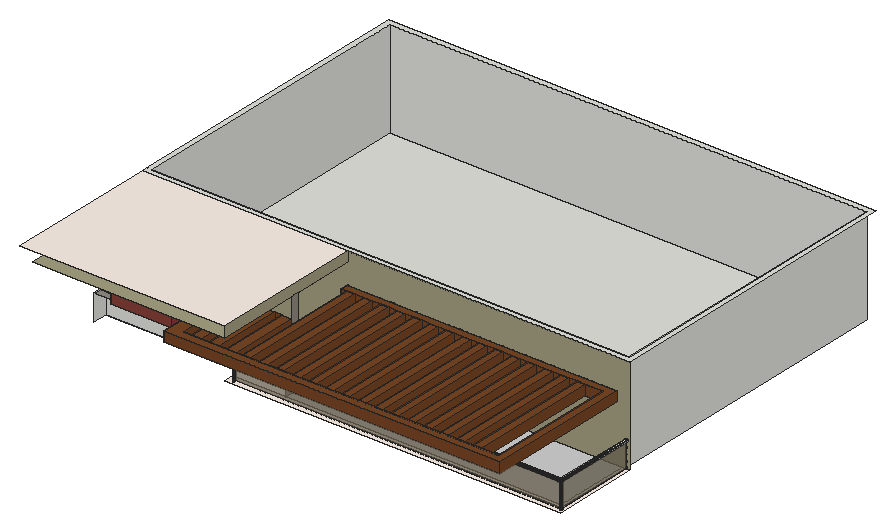
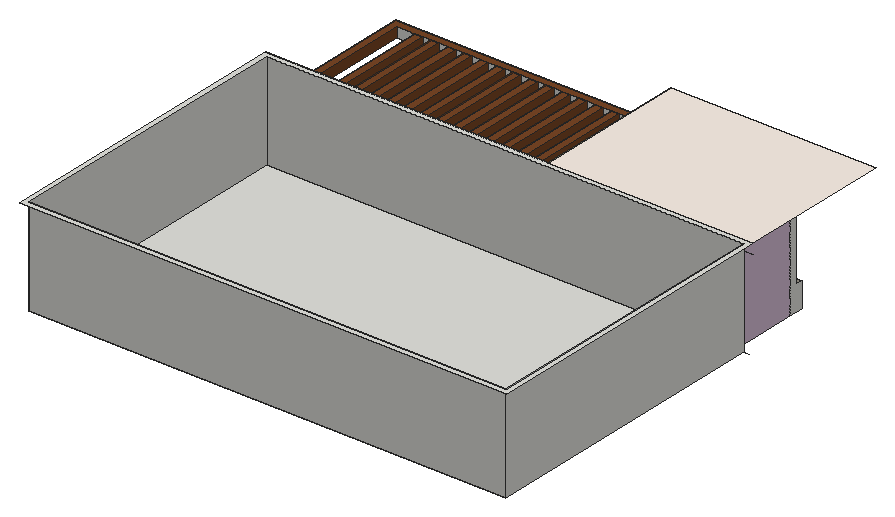
# SketchUp Ruby script. Lengths in inches.
U = 1.inch
M = Sketchup.active_model
def pt(a) = Geom::Point3d.new(a.map { |v| v * U })
def face(e, loops, mat)
  f = e.add_face(loops[0].map { |a| pt(a) })
  loops[1..].each { |l| e.add_face(l.map { |a| pt(a) }).erase! }
  f.material = f.back_material = mat if mat
  f
end
# faces: each face lists its corners as indices into pts; further lists are holes
def faces(e, pts, list, mat = nil) = list.each { |f| face(e, (f[0].is_a?(Array) ? f : [f]).map { |l| l.map { |i| pts[i] } }, mat) }
# xy, xz, yz: faces in a plane at the given z, y or x. An outline is a flat list of corners, or four numbers for a rectangle; further outlines are holes
def ring(l) = l.size == 4 ? [[l[0], l[1]], [l[2], l[1]], [l[2], l[3]], [l[0], l[3]]] : l.each_slice(2).to_a
def flat(e, list, mat, &to3) = list.each { |f| face(e, (f[0].is_a?(Array) ? f : [f]).map { |l| ring(l).map { |u, v| to3.(u, v) } }, mat) }
def xy(e, z, list, mat = nil) = flat(e, list, mat) { |x, y| [x, y, z] }
def xz(e, y, list, mat = nil) = flat(e, list, mat) { |x, z| [x, y, z] }
def yz(e, x, list, mat = nil) = flat(e, list, mat) { |y, z| [x, y, z] }
def lines(e, pts, list) = list.each { |a, b| e.add_line(pt(pts[a]), pt(pts[b])) }
# prism: a flat outline (further loops are holes) pulled along v
def prism(e, loops, v, mat = nil)
  f = face(e, loops, mat); d = Geom::Vector3d.new(v.map { |x| x * U })
  f.pushpull(f.normal.samedirection?(d) ? d.length : -d.length)
end
def box(e, o, s, mat = nil) = prism(e, [[o, [o[0] + s[0], o[1], o[2]], [o[0] + s[0], o[1] + s[1], o[2]], [o[0], o[1] + s[1], o[2]]]], [0, 0, s[2]], mat)
def at(x, y, z, deg = 0) = Geom::Transformation.translation(pt([x, y, z])) * Geom::Transformation.rotation(ORIGIN, Z_AXIS, deg.degrees)
def axes(o, x, y, z) = Geom::Transformation.new([*x, 0, *y, 0, *z, 0, *pt(o).to_a, 1])
def part(name) = M.definitions.add(name)
# library, detail: a bought-in or finely detailed component or shape, given as its bounding box
def library(name, o, s) = part(name).tap { |d| box(d.entities, o, s) }
def detail(e, o, s) = box(e.add_group.entities, o, s)
def put(e, d, t, mat = nil) = e.add_instance(d, t).tap { |i| i.material = mat if mat }
def group(e, t, mat = nil) = e.add_group.tap { |g| g.transformation = t; g.material = mat if mat }.entities
root = M.entities
M.materials.add("[0009_Linen]").color = [250, 240, 230]
M.materials.add("[0118_Thistle]").color = [216, 191, 216]
M.materials.add("[Brick Antique 01]").color = [135, 65, 58]
M.materials.add("[Carrera Marble]1").color = [207, 207, 207]
M.materials.add("[Cinder Block]").color = [145, 140, 130]
M.materials.add("[Stone Coursed Rough]").color = [165, 160, 130]
M.materials.add("[Translucent Glass Gray]").color = [128, 118, 98]
M.materials["[Translucent Glass Gray]"].alpha = 0.5
M.materials.add("[Wood Veneer 01]").color = [120, 70, 37]
xy(root,1092,[[367.55,284.98,366.77,285.08,366.05,285.38,365.43,285.86,364.95,286.48,364.65,287.2,364.55,287.98,364.65,288.76,364.95,289.48,365.43,290.1,366.05,290.58,366.77,290.88,367.55,290.98,368.32,290.88,369.05,290.58,369.67,290.1,370.14,289.48,370.44,288.76,370.55,287.98,370.44,287.2,370.14,286.48,369.67,285.86,369.05,285.38,368.32,285.08],[1134.3,284.98,1135.07,285.08,1135.8,285.38,1136.42,285.86,1136.89,286.48,1137.19,287.2,1137.3,287.98,1137.19,288.76,1136.89,289.48,1136.42,290.1,1135.8,290.58,1135.07,290.88,1133.52,290.88,1132.8,290.58,1132.18,290.1,1131.7,289.48,1131.4,288.76,1131.3,288,1131.3,287.98,1131.4,287.2,1131.7,286.48,1132.18,285.86,1132.8,285.38,1133.52,285.08],[370.55,288,1124.5,290],[1124.5,288,1131.3,290],[1131.3,288,1131.4,288.76,1131.7,289.48,1132.18,290.1,1132.8,290.58,1133.52,290.88,1133.5,290.88,1133.5,300,1124.5,300,1124.5,290,1131.3,290],
  [1133.5,290.88,1133.5,300,1135.5,300,1135.5,290.88,1135.07,290.88,1134.3,290.98,1133.52,290.88],[1133.52,290.88,1135.07,290.88,1134.3,290.98],[1124.5,300,1133.5,480],[1133.5,300,1135.5,480],[12,492,1130.5,1188]])
xy(root,1092,[[[355.9375,276,1142.5,276,1142.5,480,1135.5,480,1135.5,290.88,1135.07,290.88,1135.8,290.58,1136.42,290.1,1136.89,289.48,1137.19,288.76,1137.3,287.98,1137.19,287.2,1136.89,286.48,1136.42,285.86,1135.8,285.38,1135.07,285.08,1134.3,284.98,1133.52,285.08,1132.8,285.38,1132.18,285.86,1131.7,286.48,1131.4,287.2,1131.3,287.98,1131.3,288,370.55,288,370.55,290,1124.5,290,1124.5,300,355.9375,300],[367.55,284.98,366.77,285.08,366.05,285.38,365.43,285.86,364.95,286.48,364.65,287.2,364.55,287.98,364.65,288.76,364.95,289.48,365.43,290.1,366.05,290.58,366.77,290.88,367.55,290.98,368.32,290.88,369.05,290.58,369.67,290.1,370.14,289.48,370.44,288.76,370.55,287.98,370.44,287.2,370.14,286.48,369.67,285.86,369.05,285.38,368.32,285.08]]],"[0009_Linen]")
xy(root,1092,[[480,300,1124.5,300,1124.5,480,30,480,30,335,480,335]],"[Carrera Marble]1")
xy(root,1147.625,[[1133.5,290.88,1135.5,480]])
xy(root,1148.77,[[370.55,288,1131.29,290]])
xy(root,1152,[[30,300,78,318],[221.625,300,480,318]],"[Cinder Block]")
xy(root,1181.4,[[78,288,221.625,318]],"[Brick Antique 01]")
xy(root,1224,[[324,138,324,318,354.81,318,354.81,156,1093.05,156,1093.05,462,480,462,480,480,1111.05,480,1111.05,138],[374.32,156,398.32,318],[415.25,156,439.25,318],[456.07,156,480,318],[492.75,156,512.76,462],
  [532.5,156,552.51,462],[572.52,156,590.91,462],[610.92,156,629.3125,462],[649.32,156,667.71,462],[687.72,156,706.11,462],
  [726.12,156,744.51,462],[764.52,156,782.91,462],[802.92,156,821.3125,462],[841.32,156,859.71,462],[879.72,156,898.11,462],
  [918.12,156,936.51,462],[956.52,156,974.91,462],[994.92,156,1013.3125,462],[1033.32,156,1051.71,462]],"[Wood Veneer 01]")
xy(root,1248,[[324,138,1111.05,138,1111.05,480,480,480,480,462,1093.05,462,1093.05,156,354.81,156,354.81,318,324,318],[374.32,156,398.32,318],[415.25,156,439.25,318],[456.07,156,480,318],[492.75,156,512.76,462],
  [532.5,156,552.51,462],[572.52,156,590.91,462],[610.92,156,629.3125,462],[649.32,156,667.71,462],[687.72,156,706.11,462],
  [726.12,156,744.51,462],[764.52,156,782.91,462],[802.92,156,821.3125,462],[841.32,156,859.71,462],[879.72,156,898.11,462],
  [918.12,156,936.51,462],[956.52,156,974.91,462],[994.92,156,1013.3125,462],[1033.32,156,1051.71,462]],"[Wood Veneer 01]")
xy(root,1296,[[112.08,219.45,109.8,220.03,107.75,221.18,106.07,222.83,104.875,224.85,104.24,227.11,104.22,229.46,104.8,231.74,105.95,233.78,107.59,235.46,109.61,236.66,111.875,237.3,114.22,237.32,116.5,236.74,118.55,235.59,120.23,233.95,121.43,231.93,122.06,229.66,122.09,227.3125,121.5,225.04,120.35,222.99,118.71,221.31,116.6875,220.11,114.43,219.48],[239.58,219.45,237.3,220.03,235.25,221.18,233.57,222.83,232.375,224.85,231.74,227.11,231.72,229.46,232.3,231.74,233.45,233.78,235.09,235.46,237.11,236.66,239.375,237.3,241.72,237.32,244,236.74,246.05,235.59,247.73,233.95,248.93,231.93,249.56,229.66,249.59,227.3125,249,225.04,247.85,222.99,246.21,221.31,244.1875,220.11,241.93,219.48],[396.2,219.45,393.93,220.03,391.88,221.18,390.2,222.83,389,224.85,388.37,227.11,388.34,229.46,388.92,231.74,390.07,233.78,391.72,235.46,393.74,236.66,396,237.3,398.35,237.32,400.625,236.74,402.67,235.59,404.35,233.95,405.55,231.93,406.18,229.66,406.21,227.3125,405.63,225.04,404.48,222.99,402.84,221.31,400.8125,220.11,398.55,219.48],[30,318,480,335],[30,335,480,480]])
xy(root,1296,[[[30,120,480,318],[112.08,219.45,114.43,219.48,116.6875,220.11,118.71,221.31,120.35,222.99,121.5,225.04,122.09,227.3125,122.06,229.66,121.43,231.93,120.23,233.95,118.55,235.59,116.5,236.74,114.22,237.32,111.875,237.3,109.61,236.66,107.59,235.46,105.95,233.78,104.8,231.74,104.22,229.46,104.24,227.11,104.875,224.85,106.07,222.83,107.75,221.18,109.8,220.03],[396.2,219.45,398.55,219.48,400.8125,220.11,402.84,221.31,404.48,222.99,405.63,225.04,406.21,227.3125,406.18,229.66,405.55,231.93,404.35,233.95,402.67,235.59,400.625,236.74,398.35,237.32,396,237.3,393.74,236.66,391.72,235.46,390.07,233.78,388.92,231.74,388.34,229.46,388.37,227.11,389,224.85,390.2,222.83,391.88,221.18,393.93,220.03],[239.58,219.45,241.93,219.48,244.1875,220.11,246.21,221.31,247.85,222.99,249,225.04,249.59,227.3125,249.56,229.66,248.93,231.93,247.73,233.95,246.05,235.59,244,236.74,241.72,237.32,239.375,237.3,237.11,236.66,235.09,235.46,233.45,233.78,232.3,231.74,231.72,229.46,231.74,227.11,232.375,224.85,233.57,222.83,235.25,221.18,237.3,220.03]]],"[Stone Coursed Rough]")
xy(root,1320,[[0,480,1142.5,480,1142.5,1200,0,1200,0,492,12,492,12,1188,1130.5,1188,1130.5,492,0,492]])
xy(root,1320,[[0,120,480,480]],"[0009_Linen]")
xz(root,138,[[324,1224,1111.05,1248]],"[Wood Veneer 01]")
xz(root,156,[[354.81,1224,374.32,1248],[374.32,1224,398.32,1248],[398.32,1224,415.25,1248],[415.25,1224,439.25,1248],[439.25,1224,456.07,1248],
  [456.07,1224,480,1248],[480,1224,492.75,1248],[492.75,1224,512.76,1248],[512.76,1224,532.5,1248],[532.5,1224,552.51,1248],
  [552.51,1224,572.52,1248],[572.52,1224,590.91,1248],[590.91,1224,610.92,1248],[610.92,1224,629.3125,1248],[629.3125,1224,649.32,1248],
  [649.32,1224,667.71,1248],[667.71,1224,687.72,1248],[687.72,1224,706.11,1248],[706.11,1224,726.12,1248],[726.12,1224,744.51,1248],
  [744.51,1224,764.52,1248],[764.52,1224,782.91,1248],[782.91,1224,802.92,1248],[802.92,1224,821.3125,1248],[821.3125,1224,841.32,1248],
  [841.32,1224,859.71,1248],[859.71,1224,879.72,1248],[879.72,1224,898.11,1248],[898.11,1224,918.12,1248],[918.12,1224,936.51,1248],
  [936.51,1224,956.52,1248],[956.52,1224,974.91,1248],[974.91,1224,994.92,1248],[994.92,1224,1013.3125,1248],[1013.3125,1224,1033.32,1248],
  [1033.32,1224,1051.71,1248],[1051.71,1224,1093.05,1248]])
xz(root,288,[[78,1152,221.625,1181.4]],"[Brick Antique 01]")
xz(root,288,[[370.55,1092,1131.3,1092,1131.29,1092.02,1131.29,1148.77,370.55,1148.77]],"[Translucent Glass Gray]")
xz(root,290,[[370.55,1092,370.55,1148.77,1131.29,1148.77,1131.29,1092.02,1131.3,1092]],"[Translucent Glass Gray]")
xz(root,290.88,[[1133.5,1092,1133.52,1147.625],[1133.52,1092,1135.07,1147.625],[1135.07,1092,1135.5,1147.625]])
xz(root,290.98,[[1134.3,1149,1133.52,1149.1,1132.8,1149.4,1132.18,1149.88,1131.7,1150.5,1131.4,1151.22,1131.3,1152,1134.3,1152],[1134.3,1149,1134.3,1152,1131.3,1152,1131.4,1152.78,1131.7,1153.5,1132.18,1154.12,1132.8,1154.6,1133.52,1154.9,1134.3,1155,1135.07,1154.9,1135.8,1154.6,1136.42,1154.12,1136.89,1153.5,1137.19,1152.78,1137.3,1152,1137.19,1151.22,1136.89,1150.5,1136.42,1149.88,1135.8,1149.4,1135.07,1149.1]])
xz(root,318,[[480,1224,480.07,1248]])
xz(root,318,[[30,1152,78,1152,78,1181.4,221.625,1181.4,221.625,1152,480,1152,480,1224,324,1224,324,1248,480,1248,480,1296,30,1296]],"[Stone Coursed Rough]")
xz(root,318,[[354.81,1224,374.32,1248],[398.32,1224,415.25,1248],[439.25,1224,456.07,1248]],"[Wood Veneer 01]")
xz(root,335,[[30,1092,480,1296]])
xz(root,462,[[492.75,1224,512.76,1248],[532.5,1224,552.51,1248],[572.52,1224,590.91,1248],[610.92,1224,629.3125,1248],[649.32,1224,667.71,1248],
  [687.72,1224,706.11,1248],[726.12,1224,744.51,1248],[764.52,1224,782.91,1248],[802.92,1224,821.3125,1248],[841.32,1224,859.71,1248],
  [879.72,1224,898.11,1248],[918.12,1224,936.51,1248],[956.52,1224,974.91,1248],[994.92,1224,1013.3125,1248],[1033.32,1224,1051.71,1248]])
xz(root,462,[[480,1224,492.75,1248],[512.76,1224,532.5,1248],[552.51,1224,572.52,1248],[590.91,1224,610.92,1248],[629.3125,1224,649.32,1248],
  [667.71,1224,687.72,1248],[706.11,1224,726.12,1248],[744.51,1224,764.52,1248],[782.91,1224,802.92,1248],[821.3125,1224,841.32,1248],
  [859.71,1224,879.72,1248],[898.11,1224,918.12,1248],[936.51,1224,956.52,1248],[974.91,1224,994.92,1248],[1013.3125,1224,1033.32,1248],
  [1051.71,1224,1093.05,1248]],"[Wood Veneer 01]")
xz(root,480,[[1133.5,1092,1135.5,1147.625],[1134.3,1149,1135.07,1149.1,1135.8,1149.4,1136.42,1149.88,1136.89,1150.5,1137.19,1151.22,1137.3,1152,1137.19,1152.78,1136.89,1153.5,1136.42,1154.12,1135.8,1154.6,1135.07,1154.9,1134.3,1155,1133.52,1154.9,1132.8,1154.6,1132.18,1154.12,1131.7,1153.5,1131.4,1152.78,1131.3,1152,1131.4,1151.22,1131.7,1150.5,1132.18,1149.88,1132.8,1149.4,1133.52,1149.1],[480,1224,1111.05,1248]])
xz(root,480,[[[30,1092,1133.5,1092,1133.5,1147.625,1135.5,1147.625,1135.5,1092,1142.5,1092,1142.5,1320,480,1320,480,1296,30,1296],[480,1224,1111.05,1248],[1134.3,1149,1133.52,1149.1,1132.8,1149.4,1132.18,1149.88,1131.7,1150.5,1131.4,1151.22,1131.3,1152,1131.4,1152.78,1131.7,1153.5,1132.18,1154.12,1132.8,1154.6,1133.52,1154.9,1134.3,1155,1135.07,1154.9,1135.8,1154.6,1136.42,1154.12,1136.89,1153.5,1137.19,1152.78,1137.3,1152,1137.19,1151.22,1136.89,1150.5,1136.42,1149.88,1135.8,1149.4,1135.07,1149.1]]],"[Stone Coursed Rough]")
xz(root,492,[[12,1092,1130.5,1320]])
xz(root,1188,[[12,1092,1130.5,1320]])
yz(root,12,[[492,1092,1188,1320]])
yz(root,30,[[300,1092,335,1092,335,1296,318,1296,318,1152,300,1152]])
yz(root,30,[[335,1092,480,1296]],"[0118_Thistle]")
yz(root,78,[[288,1152,318,1181.4]],"[Brick Antique 01]")
yz(root,221.625,[[288,1152,318,1181.4]],"[Brick Antique 01]")
yz(root,324,[[138,1224,318,1248]],"[Wood Veneer 01]")
yz(root,354.81,[[156,1224,318,1248]],"[Wood Veneer 01]")
yz(root,370.55,[[288,1092,290,1148.77],[287.98,1149,287.98,1152,290.98,1152,290.88,1152.78,290.58,1153.5,290.1,1154.12,289.48,1154.6,288.76,1154.9,287.98,1155,287.2,1154.9,286.48,1154.6,285.86,1154.12,285.38,1153.5,285.08,1152.78,284.98,1152,285.08,1151.22,285.38,1150.5,285.86,1149.88,286.48,1149.4,287.2,1149.1],[287.98,1149,288.76,1149.1,289.48,1149.4,290.1,1149.88,290.58,1150.5,290.88,1151.22,290.98,1152,287.98,1152]])
yz(root,374.32,[[156,1224,318,1248]],"[Wood Veneer 01]")
yz(root,398.32,[[156,1224,318,1248]],"[Wood Veneer 01]")
yz(root,415.25,[[156,1224,318,1248]],"[Wood Veneer 01]")
yz(root,439.25,[[156,1224,318,1248]],"[Wood Veneer 01]")
yz(root,456.07,[[156,1224,318,1248]],"[Wood Veneer 01]")
yz(root,480,[[300,1092,335,1092,335,1296,318,1296,318,1152,300,1152]],"[Cinder Block]")
yz(root,480,[[120,1296,480,1320]],"[Stone Coursed Rough]")
yz(root,480,[[156,1224,318,1248],[462,1224,480,1248]],"[Wood Veneer 01]")
yz(root,492.75,[[156,1224,462,1248]],"[Wood Veneer 01]")
yz(root,512.76,[[156,1224,462,1248]],"[Wood Veneer 01]")
yz(root,532.5,[[156,1224,462,1248]],"[Wood Veneer 01]")
yz(root,552.51,[[156,1224,462,1248]],"[Wood Veneer 01]")
yz(root,572.52,[[156,1224,462,1248]],"[Wood Veneer 01]")
yz(root,590.91,[[156,1224,462,1248]],"[Wood Veneer 01]")
yz(root,610.92,[[156,1224,462,1248]],"[Wood Veneer 01]")
yz(root,629.3125,[[156,1224,462,1248]],"[Wood Veneer 01]")
yz(root,649.32,[[156,1224,462,1248]],"[Wood Veneer 01]")
yz(root,667.71,[[156,1224,462,1248]],"[Wood Veneer 01]")
yz(root,687.72,[[156,1224,462,1248]],"[Wood Veneer 01]")
yz(root,706.11,[[156,1224,462,1248]],"[Wood Veneer 01]")
yz(root,726.12,[[156,1224,462,1248]],"[Wood Veneer 01]")
yz(root,744.51,[[156,1224,462,1248]],"[Wood Veneer 01]")
yz(root,764.52,[[156,1224,462,1248]],"[Wood Veneer 01]")
yz(root,782.91,[[156,1224,462,1248]],"[Wood Veneer 01]")
yz(root,802.92,[[156,1224,462,1248]],"[Wood Veneer 01]")
yz(root,821.3125,[[156,1224,462,1248]],"[Wood Veneer 01]")
yz(root,841.32,[[156,1224,462,1248]],"[Wood Veneer 01]")
yz(root,859.71,[[156,1224,462,1248]],"[Wood Veneer 01]")
yz(root,879.72,[[156,1224,462,1248]],"[Wood Veneer 01]")
yz(root,898.11,[[156,1224,462,1248]],"[Wood Veneer 01]")
yz(root,918.12,[[156,1224,462,1248]],"[Wood Veneer 01]")
yz(root,936.51,[[156,1224,462,1248]],"[Wood Veneer 01]")
yz(root,956.52,[[156,1224,462,1248]],"[Wood Veneer 01]")
yz(root,974.91,[[156,1224,462,1248]],"[Wood Veneer 01]")
yz(root,994.92,[[156,1224,462,1248]],"[Wood Veneer 01]")
yz(root,1013.3125,[[156,1224,462,1248]],"[Wood Veneer 01]")
yz(root,1033.32,[[156,1224,462,1248]],"[Wood Veneer 01]")
yz(root,1051.71,[[156,1224,462,1248]],"[Wood Veneer 01]")
yz(root,1093.05,[[156,1224,462,1248]],"[Wood Veneer 01]")
yz(root,1111.05,[[138,1224,480,1248]],"[Wood Veneer 01]")
yz(root,1130.5,[[492,1092,1188,1320]])
yz(root,1131.29,[[288,1092.02,290,1148.77]])
yz(root,1133.5,[[290.88,1092,480,1147.625]],"[Translucent Glass Gray]")
yz(root,1135.5,[[290.88,1092,480,1147.625]],"[Translucent Glass Gray]")
p = [[366.77,285.08,1092],[367.55,284.98,1092],[367.55,284.98,1155],[366.77,285.08,1154.9],[368.32,285.08,1092],[368.32,285.08,1154.9],
  [1134.3,284.98,1092],[1133.52,285.08,1092],[1133.52,285.08,1151.22],[1134.3,284.98,1152],[1135.07,285.08,1092],[1135.07,285.08,1152.78],
  [366.05,285.38,1092],[366.05,285.38,1154.6],[369.05,285.38,1092],[369.05,285.38,1154.6],[1132.8,285.38,1092],[1132.8,285.38,1150.5],
  [1135.8,285.38,1092],[1135.8,285.38,1153.5],[365.43,285.86,1092],[365.43,285.86,1154.12],[369.67,285.86,1092],[369.67,285.86,1154.12],
  [1132.18,285.86,1092],[1132.18,285.86,1149.88],[1136.42,285.86,1092],[1136.42,285.86,1154.12],[364.95,286.48,1092],[364.95,286.48,1153.5],
  [370.14,286.48,1092],[370.14,286.48,1153.5],[1131.7,286.48,1092],[1131.7,286.48,1149.4],[1136.89,286.48,1092],[1136.89,286.48,1154.6],
  [364.65,287.2,1092],[364.65,287.2,1152.78],[370.44,287.2,1092],[370.44,287.2,1152.78],[1131.4,287.2,1092],[1131.4,287.2,1149.1],
  [1137.19,287.2,1092],[1137.19,287.2,1154.9],[364.55,287.98,1092],[364.55,287.98,1152],[370.55,287.98,1092],[370.55,287.98,1149],
  [370.55,287.98,1152],[1131.3,287.98,1092],[1131.3,287.98,1149],[1137.3,287.98,1092],[1137.3,287.98,1155],[364.65,288.76,1092],
  [364.65,288.76,1151.22],[370.44,288.76,1092],[370.44,288.76,1151.22],[1131.3,288,1092],[1131.4,288.76,1092],[1131.4,288.76,1149.1],
  [1131.29,288,1092.02],[1131.3,290,1092],[1131.29,290,1092.02],[1137.19,288.76,1092],[1137.19,288.76,1154.9],[364.95,289.48,1092],
  [364.95,289.48,1150.5],[370.14,289.48,1092],[370.14,289.48,1150.5],[1131.7,289.48,1092],[1131.7,289.48,1149.4],[1136.89,289.48,1092],
  [1136.89,289.48,1154.6],[365.43,290.1,1092],[365.43,290.1,1149.88],[369.67,290.1,1092],[369.67,290.1,1149.88],[1132.18,290.1,1092],
  [1132.18,290.1,1149.88],[1136.42,290.1,1092],[1136.42,290.1,1154.12],[366.05,290.58,1092],[366.05,290.58,1149.4],[369.05,290.58,1092],
  [369.05,290.58,1149.4],[1132.8,290.58,1092],[1132.8,290.58,1150.5],[1135.8,290.58,1092],[1135.8,290.58,1153.5],[366.77,290.88,1092],
  [366.77,290.88,1149.1],[368.32,290.88,1092],[368.32,290.88,1149.1],[1133.52,290.88,1092],[1133.52,290.88,1147.625],[1133.52,290.88,1151.22],
  [1135.07,290.88,1092],[1135.07,290.88,1152.78],[1135.07,290.88,1147.625],[367.55,290.98,1092],[367.55,290.98,1149],[1134.3,290.98,1092],
  [1134.3,290.98,1149],[1134.3,290.98,1152],[370.55,287.2,1149.1],[370.55,288.76,1149.1],[366.77,300,1149.1],[367.55,300,1149],
  [368.32,300,1149.1],[1134.3,480,1149],[1133.52,480,1149.1],[1133.52,290.98,1149.1],[1135.07,480,1149.1],[1135.07,290.98,1149.1],
  [370.55,286.48,1149.4],[370.55,289.48,1149.4],[366.05,300,1149.4],[369.05,300,1149.4],[1132.8,480,1149.4],[1132.8,290.98,1149.4],
  [1135.8,480,1149.4],[1135.8,290.98,1149.4],[370.55,285.86,1149.88],[370.55,290.1,1149.88],[365.43,300,1149.88],[369.67,300,1149.88],
  [1132.18,480,1149.88],[1132.18,290.98,1149.88],[1136.42,480,1149.88],[1136.42,290.98,1149.88],[370.55,285.38,1150.5],[364.95,300,1150.5],
  [370.14,300,1150.5],[370.55,290.58,1150.5],[1131.7,480,1150.5],[1131.7,290.98,1150.5],[1136.89,480,1150.5],[1136.89,290.98,1150.5],
  [370.55,285.08,1151.22],[364.65,300,1151.22],[370.44,300,1151.22],[370.55,290.88,1151.22],[1131.4,480,1151.22],[1131.4,290.98,1151.22],
  [1137.19,480,1151.22],[1137.19,290.98,1151.22],[370.55,284.98,1152],[364.55,300,1152],[370.55,300,1152],[370.55,290.98,1152],
  [1131.3,290.98,1152],[1131.3,480,1152],[1137.3,480,1152],[1137.3,290.98,1152],[370.55,285.08,1152.78],[364.65,300,1152.78],
  [370.44,300,1152.78],[370.55,290.88,1152.78],[1131.4,480,1152.78],[1131.4,290.98,1152.78],[1137.19,480,1152.78],[1137.19,290.98,1152.78],
  [370.55,285.38,1153.5],[364.95,300,1153.5],[370.14,300,1153.5],[370.55,290.58,1153.5],[1131.7,480,1153.5],[1131.7,290.98,1153.5],
  [1136.89,480,1153.5],[1136.89,290.98,1153.5],[370.55,285.86,1154.12],[365.43,300,1154.12],[369.67,300,1154.12],[370.55,290.1,1154.12],
  [1132.18,480,1154.12],[1132.18,290.98,1154.12],[1136.42,480,1154.12],[1136.42,290.98,1154.12],[366.05,300,1154.6],[369.05,300,1154.6],
  [370.55,286.48,1154.6],[370.55,289.48,1154.6],[1132.8,480,1154.6],[1132.8,290.98,1154.6],[1135.8,480,1154.6],[1135.8,290.98,1154.6],
  [366.77,300,1154.9],[368.32,300,1154.9],[370.55,287.2,1154.9],[370.55,288.76,1154.9],[1133.52,480,1154.9],[1133.52,290.98,1154.9],
  [1135.07,480,1154.9],[1135.07,290.98,1154.9],[367.55,300,1155],[370.55,287.98,1155],[1134.3,480,1155],[1134.3,290.98,1155],
  [0,492,1092],[12,492,1092],[30,480,1296],[0,480,1296],[1134.3,287.98,1092],[1134.3,287.98,1152],
  [367.55,287.98,1092],[367.55,287.98,1152],[367.55,300,1152],[1134.3,480,1152]]
faces(root,p,[[0,1,2,3],[1,4,5,2],[6,7,8,9],[10,6,9,11],[12,0,3,13],[4,14,15,5],[7,16,17,8],[18,10,11,19],
  [20,12,13,21],[14,22,23,15],[16,24,25,17],[26,18,19,27],[28,20,21,29],[22,30,31,23],[24,32,33,25],[34,26,27,35],
  [36,28,29,37],[30,38,39,31],[32,40,41,33],[42,34,35,43],[44,36,37,45],[38,46,47,48,39],[40,49,50,41],[51,42,43,52],
  [53,44,45,54],[46,55,56,48,47],[57,58,59,50,49],[60,57,61,62],[63,51,52,64],[65,53,54,66],[55,67,68,56],[58,69,70,59],
  [71,63,64,72],[73,65,66,74],[67,75,76,68],[69,77,78,70],[79,71,72,80],[81,73,74,82],[75,83,84,76],[77,85,86,78],
  [87,79,80,88],[89,81,82,90],[83,91,92,84],[85,93,94,95,86],[96,87,88,97,98],[99,89,90,100],[91,99,100,92],[93,101,102,103,95,94],
  [101,96,98,97,103,102],[41,50,47,104],[50,59,105,47],[100,90,106,107],[92,100,107,108],[109,110,111,102],[112,109,102,113],[33,41,104,114],
  [59,70,115,105],[90,82,116,106],[84,92,108,117],[110,118,119,111],[120,112,113,121],[25,33,114,122],[70,78,123,115],[82,74,124,116],
  [76,84,117,125],[118,126,127,119],[128,120,121,129],[17,25,122,130],[74,66,131,124],[68,76,125,132],[78,86,133,123],[126,134,135,127],
  [136,128,129,137],[8,17,130,138],[66,54,139,131],[56,68,132,140],[86,95,141,133],[134,142,143,135],[144,136,137,145],[9,8,138,146],
  [54,45,147,139],[48,56,140,148,149],[95,103,150,149,141],[142,151,150,143],[152,144,145,153],[11,9,146,154],[45,37,155,147],[39,48,149,148,156],
  [103,97,157,149,150],[151,158,159,150],[160,152,153,161],[19,11,154,162],[37,29,163,155],[31,39,156,164],[97,88,165,157],[158,166,167,159],
  [168,160,161,169],[27,19,162,170],[29,21,171,163],[23,31,164,172],[88,80,173,165],[166,174,175,167],[176,168,169,177],[21,13,178,171],
  [15,23,172,179],[35,27,170,180],[80,72,181,173],[174,182,183,175],[184,176,177,185],[13,3,186,178],[5,15,179,187],[43,35,180,188],
  [72,64,189,181],[182,190,191,183],[192,184,185,193],[3,2,194,186],[2,5,187,194],[52,43,188,195],[64,52,195,189],[190,196,197,191],
  [196,192,193,197]])
lines(root,p,[[198,199],[200,201],[202,203],[203,103],[204,205],[205,206],[205,48],[48,203],[103,207]])
